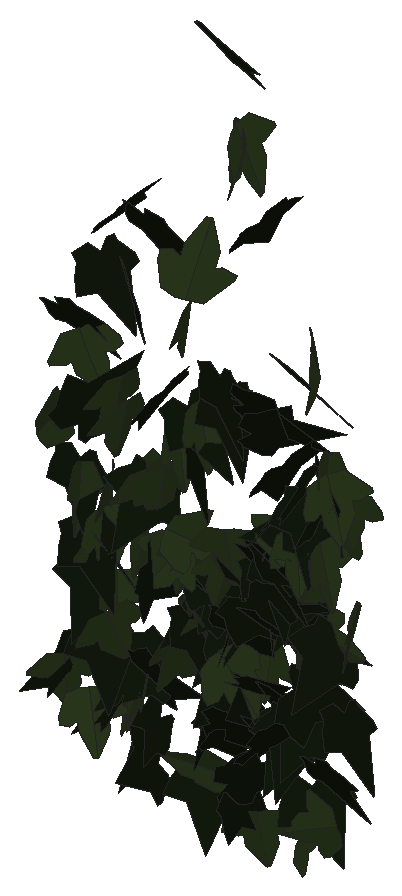
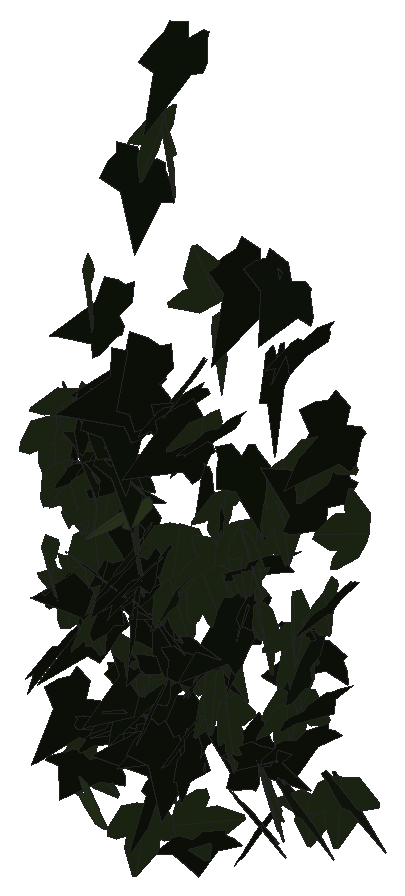
# SketchUp Ruby script. Lengths in inches.
U = 1.inch
M = Sketchup.active_model
def pt(a) = Geom::Point3d.new(a.map { |v| v * U })
def face(e, loops, mat)
  f = e.add_face(loops[0].map { |a| pt(a) })
  loops[1..].each { |l| e.add_face(l.map { |a| pt(a) }).erase! }
  f.material = f.back_material = mat if mat
  f
end
# faces: each face lists its corners as indices into pts; further lists are holes
def faces(e, pts, list, mat = nil) = list.each { |f| face(e, (f[0].is_a?(Array) ? f : [f]).map { |l| l.map { |i| pts[i] } }, mat) }
# xy, xz, yz: faces in a plane at the given z, y or x. An outline is a flat list of corners, or four numbers for a rectangle; further outlines are holes
def ring(l) = l.size == 4 ? [[l[0], l[1]], [l[2], l[1]], [l[2], l[3]], [l[0], l[3]]] : l.each_slice(2).to_a
def flat(e, list, mat, &to3) = list.each { |f| face(e, (f[0].is_a?(Array) ? f : [f]).map { |l| ring(l).map { |u, v| to3.(u, v) } }, mat) }
def xy(e, z, list, mat = nil) = flat(e, list, mat) { |x, y| [x, y, z] }
def xz(e, y, list, mat = nil) = flat(e, list, mat) { |x, z| [x, y, z] }
def yz(e, x, list, mat = nil) = flat(e, list, mat) { |y, z| [x, y, z] }
def lines(e, pts, list) = list.each { |a, b| e.add_line(pt(pts[a]), pt(pts[b])) }
# prism: a flat outline (further loops are holes) pulled along v
def prism(e, loops, v, mat = nil)
  f = face(e, loops, mat); d = Geom::Vector3d.new(v.map { |x| x * U })
  f.pushpull(f.normal.samedirection?(d) ? d.length : -d.length)
end
def box(e, o, s, mat = nil) = prism(e, [[o, [o[0] + s[0], o[1], o[2]], [o[0] + s[0], o[1] + s[1], o[2]], [o[0], o[1] + s[1], o[2]]]], [0, 0, s[2]], mat)
def at(x, y, z, deg = 0) = Geom::Transformation.translation(pt([x, y, z])) * Geom::Transformation.rotation(ORIGIN, Z_AXIS, deg.degrees)
def axes(o, x, y, z) = Geom::Transformation.new([*x, 0, *y, 0, *z, 0, *pt(o).to_a, 1])
def part(name) = M.definitions.add(name)
# library, detail: a bought-in or finely detailed component or shape, given as its bounding box
def library(name, o, s) = part(name).tap { |d| box(d.entities, o, s) }
def detail(e, o, s) = box(e.add_group.entities, o, s)
def put(e, d, t, mat = nil) = e.add_instance(d, t).tap { |i| i.material = mat if mat }
def group(e, t, mat = nil) = e.add_group.tap { |g| g.transformation = t; g.material = mat if mat }.entities
root = M.entities
M.materials.add("efeu1").color = [18, 25, 13]
M.materials.add("efeu2").color = [43, 57, 29]
c1 = part("ivyleaf_9")
p = [[1.54,2.16,1.25],[1.36,2.04,1.19],[-0.21,0.99,0.68],[-0.71,1.11,0.82],[-0.85,0.86,0.67],[-0.8,0.17,0.21],
  [-0.9,-0.01,0.1],[-0.67,-0.16,-0.02],[-0.08,-0.08,-0.05],[-0.03,-0.6,-0.4],[0.65,-0.88,-0.66],[0.83,-0.6,-0.49],
  [1.29,-0.42,-0.43],[1.8125,-0.07,-0.26],[1.21,0.44,0.15]]
faces(c1.entities,p,[[0,1,2,3,4,5,6,7,8,9,10,11,12,13,14]],"efeu1")
c2 = part("ivyleaf_10")
p = [[0,0.5,-0.03],[-0.0625,2.02,-0.43],[-0.19,2.01,-0.46],[-0.54,1.05,-0.29],[-0.52,0.625,-0.18],[-0.83,0.76,-0.28],
  [-1.16,0.64,-0.33],[-1.15,0.33,-0.24],[-0.77,-0.39,0.02],[-0.3,-0.51,0.16],[0.04,-0.48,0.23],[-0.02,2.01,-0.4375],
  [-0.06,2.01,-0.43],[0.04,-0.49,0.23],[0.67,-0.49,0.14],[1.38,0.36,-0.2],[1.375,0.51,-0.24],[0.81,0.65,-0.19],
  [0.62,0.59,-0.15],[0.6,1.09,-0.28],[0.5,1.23,-0.31]]
faces(c2.entities,p,[[0,1,2,3,4,5,6,7,8,9,10],[11,12,0,13,14,15,16,17,18,19,20]],"efeu2")
put(root,c1,axes([577.06,128.89,247.8],[-0.79782,0.64432,0.02333],[-0.05599,-0.03226,-1.02374],[-0.64231,-0.79751,0.06026]))
put(root,c2,axes([576.92,128.93,247.56],[-0.7328,-0.71537,-0.04037],[0.0378,0.01907,-1.02401],[0.71551,-0.73367,0.01274]))
put(root,c2,axes([576.88,128.08,257.89],[0.12693,-0.46512,1.05499],[-0.17832,1.04067,0.48026],[-1.1391,-0.21474,0.04237]))
put(root,c1,axes([576.91,129.79,255.57],[0.15146,-1.05206,0.06443],[0.00604,-0.06422,-1.0629],[1.05401,0.15154,-0.00316]))
put(root,c1,axes([576.97,128.67,262.52],[1.0872,0.15846,-0.03375],[-0.03824,0.02847,-1.09817],[-0.15743,1.08735,0.03367]))
put(root,c2,axes([577.51,129.17,255.4],[-0.09441,0.97241,-0.40538],[-0.04382,-0.41028,-0.97395],[-1.05261,-0.07014,0.0769]))
put(root,c1,axes([577.68,129.9375,251.1],[-0.32025,-0.94857,0.31634],[0.01052,-0.33535,-0.99491],[0.99987,-0.30029,0.11179]))
put(root,c2,axes([577.79,128.96,261.32],[-0.6989,-0.79219,-0.30752],[0.4449,-0.00187,-1.0063],[0.72401,-0.76356,0.32152]))
put(root,c2,axes([578.26,129.79,255.1],[0.37186,-0.92594,-0.35762],[-0.00755,0.37924,-0.98978],[0.99258,0.34978,0.12645]))
put(root,c2,axes([578.33,129.57,252.96],[-0.17488,-1.04729,0.05785],[0.19474,-0.09005,-1.0415],[1.03065,-0.16069,0.20661]))
put(root,c1,axes([577.74,129.77,252.8],[0.73564,-0.65,0.38792],[0.27873,-0.27032,-0.98152],[0.70377,0.78649,-0.01675]))
put(root,c1,axes([577.98,129.01,253.44],[-0.45566,-0.41074,-0.91799],[0.81737,0.43592,-0.60076],[0.58593,-0.92752,0.12417]))
put(root,c2,axes([578.2,128.71,246.47],[0.89283,0.43868,0.24577],[0.23293,0.08302,-0.9944],[-0.44563,0.92231,-0.02738]))
put(root,c1,axes([579.09,129.2,246.96],[-0.84178,0.56961,-0.05662],[0.04864,-0.02914,-1.01639],[-0.57035,-0.84318,-0.00312]))
put(root,c2,axes([578.53,129.26,253.82],[0.29311,1.02348,0.03769],[-0.06124,0.05665,-1.06202],[-1.02234,0.29004,0.07442]))
put(root,c1,axes([578.3125,128.08,258.54],[-0.13621,-0.13847,1.15186],[0.95976,0.63812,0.1902],[-0.65179,0.96858,0.03936]))
put(root,c2,axes([578.56,129.98,250.9],[0.095,1.01006,-0.29537],[0.00689,-0.29716,-1.01397],[-1.05234,0.08924,-0.0333]))
put(root,c1,axes([578.57,129.33,249.22],[-0.18032,-1.0131,-0.20221],[0.07323,0.19222,-1.02834],[1.03049,-0.19094,0.03769]))
put(root,c2,axes([579.3125,129.29,258.75],[-0.17827,-1.06893,-0.03979],[-0.02023,0.0437,-1.08336],[1.06948,-0.17735,-0.02713]))
put(root,c2,axes([579.32,129.06,259.875],[-0.15944,-1.08106,0.02862],[0.00294,-0.02937,-1.09273],[1.08144,-0.1593,0.00719]))
put(root,c1,axes([578.84,128.67,265.34],[0.30481,-0.93347,-0.48956],[-0.09061,0.48453,-0.98029],[1.05016,0.31275,0.05752]))
put(root,c2,axes([579.26,128.62,250.3],[-0.47944,-0.90072,-0.37557],[0.20089,0.31839,-1.02004],[0.95498,-0.51917,0.02602]))
put(root,c1,axes([579.86,128.95,264.28],[0.45779,0.08634,-1.10755],[-1.10437,0.16518,-0.4436],[0.12039,1.187,0.14229]))
put(root,c1,axes([579.61,128.51,267.49],[0.29425,0.92645,0.52974],[-0.03106,0.55671,-0.95636],[-1.06676,0.23934,0.17397]))
put(root,c2,axes([579.47,129.82,247.13],[0.75626,-0.72269,0.01223],[-0.00289,-0.02073,-1.04591],[0.72279,0.75608,-0.01699]))
put(root,c2,axes([579.7,129.77,247.4375],[0.80947,-0.66459,0.01205],[0.00806,-0.00917,-1.04734],[0.66465,0.8095,-0.00197]))
put(root,c1,axes([580.34,130.08,248.33],[-0.92376,-0.37392,0.24336],[-0.22806,-0.08518,-0.99654],[0.38344,-0.95147,-0.00642]))
put(root,c2,axes([580.13,129.28,253.89],[0.85893,-0.58825,-0.24217],[-0.0937,0.28548,-1.02575],[0.62921,0.84552,0.17785]))
put(root,c1,axes([580.53,129.82,245.99],[-0.93245,0.00042,-0.43465],[0.43123,-0.12795,-0.92524],[-0.05444,-1.0208,0.11579]))
put(root,c1,axes([580.58,129.61,255.86],[-0.6201,-0.82302,0.29027],[0.01548,-0.3664,-1.00581],[0.87257,-0.57839,0.22412]))
put(root,c1,axes([581.04,129.39,260.05],[-0.33209,1.01356,-0.1565],[0.02718,-0.15574,-1.06634],[-1.02521,-0.33244,0.02243]))
put(root,c1,axes([580.62,129.58,244.3125],[-0.28381,-0.40205,0.91877],[-0.15346,-0.92619,-0.4527],[0.99107,-0.25855,0.193]))
put(root,c2,axes([580.82,129.35,256.7],[0.8085,-0.67201,-0.18203],[-0.12031,0.1399,-1.05088],[0.68575,0.81685,0.03024]))
put(root,c2,axes([580.85,128.8,256.76],[-0.39099,-0.992,-0.26862],[0.09799,0.25011,-1.06627],[1.02304,-0.40308,-0.00053]))
put(root,c1,axes([580.24,129.65,247.81],[0.36484,-0.29991,0.91578],[0.74932,-0.52741,-0.47124],[0.60591,0.83283,0.03135]))
put(root,c1,axes([580.86,128.76,267.54],[1.20109,0.17587,-0.44977],[-0.44958,-0.0331,-1.21352],[-0.17636,1.28212,0.03037]))
put(root,c2,axes([581.18,129.99,249.74],[0.1389,-1.04108,-0.08736],[0.02626,0.09158,-1.04962],[1.04441,0.13615,0.03801]))
put(root,c1,axes([581.3125,128.31,253.44],[0.25462,-0.22787,-1.11533],[-0.84985,0.72234,-0.34159],[0.75739,0.88713,-0.00834]))
put(root,c2,axes([581.29,129.17,256.69],[-0.40381,-0.99757,-0.03403],[-0.00365,0.03818,-1.07606],[0.99815,-0.40344,-0.0177]))
put(root,c1,axes([580.98,129.7,253.25],[1.10341,-0.18849,-0.00836],[-0.00859,-0.00064,-1.1194],[0.18848,1.10345,-0.00208]))
put(root,c2,axes([581.65,129.71,258.41],[0.09464,1.06557,-0.0634],[-0.01788,-0.06206,-1.06969],[-1.0673,0.09553,0.0123]))
put(root,c2,axes([582.14,128.71,254.09],[0.91405,0.05653,-0.56273],[-0.56544,0.11302,-0.9071],[0.01146,1.06741,0.12585]))
put(root,c2,axes([582.1,129.82,250.87],[-0.90474,0.44109,0.26771],[-0.27617,0.0425,-1.00335],[-0.43584,-0.94256,0.08004]))
put(root,c2,axes([583.01,130.03,244.6],[-0.30018,0.16608,-0.97809],[-0.98382,-0.18152,0.27112],[-0.12785,1.00689,0.21021]))
put(root,c2,axes([582.55,129.51,254.28],[-0.28991,-0.98191,0.31894],[-0.04548,-0.31881,-1.02284],[1.03141,-0.29006,0.04455]))
put(root,c1,axes([582.99,130.12,251.95],[-1.03943,-0.02307,0.01489],[-0.01517,0.01257,-1.03961],[0.02289,-1.03946,-0.01291]))
put(root,c2,axes([582.62,128.57,250.34],[-0.14334,-0.9298,-0.828],[0.17778,0.80964,-0.93996],[1.23228,-0.22496,0.03929]))
put(root,c2,axes([582.78,128.67,264.4],[0.41347,-1.00666,-0.21323],[0.00175,0.23049,-1.08474],[1.02899,0.40411,0.08753]))
put(root,c1,axes([582.51,130.36,244.21],[-0.41387,-0.8742,-0.30009],[0.212,0.23025,-0.96312],[0.89963,-0.45643,0.08891]))
put(root,c1,axes([582.29,129.56,258.34],[-0.27173,-0.01761,-1.03792],[1.03789,0.01554,-0.27199],[0.0195,-1.07279,0.01309]))
put(root,c1,axes([582.5,129.3,251.09],[0.42187,-0.94909,-0.08441],[-0.03216,0.07808,-1.03862],[0.95229,0.42308,0.00232]))
put(root,c2,axes([582.54,128.58,254.9375],[0.33371,0.3441,0.95667],[0.47417,0.838,-0.46681],[-0.89933,0.56952,0.10886]))
put(root,c1,axes([582.89,130.375,247.69],[-0.1635,0.09515,-1.0236],[0.80095,-0.63795,-0.18724],[-0.64444,-0.81702,0.02699]))
put(root,c1,axes([583.1,130.58,247.94],[-0.1825,-0.64065,0.78184],[-0.07454,-0.78379,-0.65964],[1.00805,-0.17394,0.09277]))
put(root,c2,axes([583.1,128.43,265.83],[0.73989,0.84599,-0.48301],[0.3262,0.35637,1.12384],[0.91793,-0.80854,-0.01004]))
put(root,c1,axes([582.86,128.73,260.29],[0.40345,-0.89232,-0.45673],[0.02712,0.50187,-0.95656],[1.00205,0.34569,0.20978]))
put(root,c2,axes([583.73,129.98,253.85],[-0.28699,-0.98923,0.23334],[-0.01998,-0.23693,-1.02901],[1.01618,-0.28404,0.04567]))
put(root,c2,axes([583.5,128.71,260.25],[0.14802,1.07471,0.00521],[-0.00575,0.00605,-1.08483],[-1.0747,0.14799,0.00652]))
put(root,c1,axes([584.15,130.3125,251.17],[-0.89848,-0.50276,0.04313],[-0.04288,-0.0117,-1.02953],[0.50278,-0.89944,-0.01072]))
put(root,c1,axes([583.625,129,259.91],[0.55669,0.6289,0.69898],[0.47305,0.51468,-0.83983],[-0.81259,0.73046,-0.01005]))
put(root,c1,axes([584.13,128.8125,275.97],[1.01169,0.35803,-0.70253],[-0.78327,0.32487,-0.96239],[-0.09069,1.18807,0.47487]))
put(root,c1,axes([584.33,129.3,247.21],[0.27982,0.98286,-0.06512],[-0.03251,-0.05844,-1.02181],[-0.98448,0.28129,0.01523]))
put(root,c1,axes([584.13,130.39,252.45],[-0.39958,0.05698,-0.9592],[0.8047,-0.54789,-0.36777],[-0.52514,-0.88292,0.16631]))
put(root,c1,axes([583.68,129.97,253.89],[0.73557,-0.75627,0.08125],[0.13031,0.01394,-1.04997],[0.74938,0.73991,0.10283]))
put(root,c2,axes([584.45,128.96,255.35],[-0.97093,-0.47407,-0.06035],[0.05132,0.03245,-1.08047],[0.47513,-0.97227,-0.00663]))
put(root,c1,axes([584.01,129.09,261.76],[0.45563,-0.97493,0.12419],[0.04159,-0.11764,-1.07608],[0.98193,0.45737,-0.01205]))
put(root,c1,axes([584.58,130.32,252.67],[-0.88058,-0.12919,-0.52249],[0.53236,-0.0616,-0.88199],[0.07923,-1.02206,0.1192]))
put(root,c1,axes([583.98,128.69,247.65],[0.99081,0.19349,0.34196],[0.33382,0.07469,-1.00948],[-0.20722,1.04549,0.00883]))
put(root,c1,axes([584.29,129.3,261.07],[0.11435,-1.05858,-0.20086],[-0.0339,0.19836,-1.06467],[1.07694,0.11865,-0.01218]))
put(root,c2,axes([584.48,128.89,250.08],[0.55426,0.87957,0.5498],[0.22772,0.50497,-1.03743],[-1.01196,0.59539,0.06767]))
put(root,c2,axes([585.21,128.69,271.97],[0.50559,-0.82129,-0.7829],[-0.41238,0.66549,-0.96443],[1.05707,0.65243,-0.00178]))
put(root,c1,axes([584.81,130.19,248.22],[-0.12339,-0.38649,0.96478],[-0.11085,-0.96112,-0.3992],[1.03339,-0.14925,0.07238]))
put(root,c1,axes([585.17,128.61,245.24],[0.31343,-0.39065,-0.97171],[-0.61076,0.75578,-0.50085],[0.85077,0.68649,-0.00157]))
put(root,c1,axes([585.07,128.625,252.47],[1.05621,0.4368,-0.28002],[-0.25891,-0.10666,-1.14297],[-0.44963,1.08748,0.00037]))
put(root,c2,axes([585.27,128.85,272.35],[-0.12275,1.16093,0.32077],[-0.05871,0.31628,-1.16715],[-1.20299,-0.13389,0.02423]))
put(root,c2,axes([585.52,129.52,243.69],[-0.86853,-0.58891,-0.0854],[0.07563,0.04063,-1.04933],[0.59024,-0.87177,0.00879]))
put(root,c2,axes([585.51,129.94,255.35],[0.62998,-0.85151,-0.01828],[0.07467,0.07787,-1.05387],[0.84843,0.62541,0.10632]))
put(root,c1,axes([585.54,129.14,249.6],[0.92485,0.35972,-0.30435],[-0.36334,0.11756,-0.96516],[-0.30002,0.96651,0.23066]))
put(root,c1,axes([585.09,130.48,252.79],[0.06626,-0.00026,-1.0344],[0.9848,-0.3171,0.06317],[-0.31646,-0.98682,-0.02002]))
put(root,c1,axes([585.17,129.07,249.4375],[1.0613,0.27677,0.27272],[0.20706,0.26839,-1.07816],[-0.32879,1.06241,0.20132]))
put(root,c1,axes([585.3125,130.11,253.88],[0.34777,-0.96398,-0.24228],[-0.0021,0.25597,-1.02145],[0.99395,0.33783,0.08261]))
put(root,c2,axes([585.68,129.8,250.65],[1.01778,-0.15175,-0.03007],[-0.00333,0.17855,-1.01386],[0.15466,1.00245,0.17603]))
put(root,c1,axes([585.41,127.97,245.89],[0.4295,0.2747,0.93557],[0.79359,0.49551,-0.50981],[-0.56654,0.90235,-0.00486]))
put(root,c1,axes([585.48,129.09,255.1875],[1.04904,0.08714,0.11459],[0.11593,-0.0117,-1.05244],[-0.08534,1.05521,-0.02114]))
put(root,c1,axes([585.68,129.55,254.78],[1.05542,0.1427,-0.16912],[-0.16501,-0.0416,-1.06485],[-0.14743,1.06807,-0.01888]))
put(root,c1,axes([585.85,130.26,254.16],[0.14809,-1.02702,0.11184],[0.01306,-0.11111,-1.03764],[1.03301,0.14864,-0.00292]))
put(root,c1,axes([586.59,128.19,269.64],[0.06067,1.11423,0.15178],[0.00548,0.1517,-1.11587],[-1.1245,0.06086,0.00275]))
put(root,c1,axes([585.87,128.55,253.4],[-0.09701,-0.13846,-1.08358],[0.42376,0.99789,-0.16545],[1.00685,-0.43333,-0.03477]))
put(root,c1,axes([585.91,129.46,254.89],[0.70056,-0.78526,0.03083],[0.05944,0.01176,-1.05105],[0.78361,0.70114,0.05216]))
put(root,c1,axes([585.59,128.75,261.33],[1.01534,-0.20811,0.64502],[0.6316,-0.13089,-1.03644],[0.24585,1.19575,-0.00119]))
put(root,c1,axes([586.45,130.46,247.49],[-0.25145,-0.98898,0.18704],[-0.00311,-0.19202,-1.01951],[1.0065,-0.24767,0.04357]))
put(root,c1,axes([586.48,128,247.79],[0.47519,0.66369,0.75251],[0.32822,0.684,-0.81053],[-0.94817,0.5694,0.09655]))
put(root,c2,axes([586.13,129.09,256.16],[0.75807,-0.66906,-0.29363],[0.62188,0.81294,-0.24683],[0.38357,0.00428,0.98051]))
put(root,c1,axes([586.74,130.41,247.8],[-0.7456,-0.72291,-0.02914],[0.14093,-0.10407,-1.02405],[0.70964,-0.73888,0.17275]))
put(root,c1,axes([587.21,128.45,257.47],[-0.17083,1.00321,0.31999],[-0.14901,0.29788,-1.01344],[-1.04241,-0.20698,0.09243]))
put(root,c1,axes([586.13,128.5,260.56],[0.75911,0.30787,0.82494],[0.74037,0.36638,-0.81803],[-0.47661,1.0595,0.04316]))
put(root,c1,axes([587.4,128.53,259.6],[-0.04557,1.09241,-0.10476],[0.02756,-0.10368,-1.09312],[-1.09708,-0.04798,-0.02311]))
put(root,c1,axes([587.41,130.5,253.88],[-0.95436,-0.18504,-0.36514],[0.39814,-0.20428,-0.93708],[0.09515,-1.00119,0.25868]))
put(root,c2,axes([587.65,129.78,254.41],[-0.97496,0.00075,0.3707],[-0.37003,-0.06486,-0.97306],[0.02235,-1.04104,0.0609]))
put(root,c2,axes([587.31,129.45,256.04],[0.451,0.94161,-0.02503],[-0.01393,-0.02108,-1.04404],[-0.94184,0.4512,0.00346]))
put(root,c1,axes([588.22,129.6875,256.84],[-0.21286,-0.32121,-0.99616],[-0.55577,-0.82672,0.38533],[-0.88692,0.59514,-0.00238]))
put(root,c1,axes([588.08,128.85,258.8],[-0.74346,0.73663,-0.22142],[0.08207,-0.23021,-1.04146],[-0.76479,-0.74078,0.10347]))
put(root,c2,axes([587.57,129.86,251.55],[-0.09183,0.939,-0.42122],[0.0128,-0.42182,-0.94312],[-1.02907,-0.08904,0.02585]))
put(root,c2,axes([587.32,129.88,243.31],[0.31596,-0.77769,-0.65248],[0.56347,-0.43408,0.79022],[-0.84442,-0.58064,0.28316]))
put(root,c2,axes([588.45,129.54,251.76],[-0.89327,-0.10422,0.56888],[-0.53986,-0.2252,-0.88896],[0.20745,-1.03482,0.13617]))
put(root,c1,axes([587.26,129.7,252.49],[0.22627,0.09525,-1.03432],[0.80175,0.65699,0.2359],[0.66037,-0.83029,0.068]))
put(root,c2,axes([587.64,129.78,256.12],[-0.13818,0.15546,-1.04467],[0.46748,-0.93575,-0.20109],[-0.94708,-0.48457,0.05316]))
put(root,c1,axes([587.66,129.99,245.53],[-0.24405,-0.71089,-0.71488],[0.47684,0.56666,-0.72629],[0.88828,-0.49951,0.19347]))
put(root,c1,axes([587.35,128.84,263.54],[0.90915,-0.54833,0.2968],[0.33262,-0.01732,-1.05089],[0.52737,0.95621,0.15116]))
put(root,c1,axes([587.95,129.63,257.61],[-0.18978,-1.04973,-0.09161],[0.00893,0.09148,-1.06672],[1.05368,-0.18984,-0.00745]))
put(root,c2,axes([588.97,129.11,244.82],[-0.39798,0.03149,0.95846],[-0.93561,-0.24041,-0.3806],[0.21039,-1.00957,0.12053]))
put(root,c1,axes([588.07,128.46,250.47],[0.44067,-0.05563,-1.07306],[-0.43966,1.04893,-0.23493],[0.98043,0.49538,0.37695]))
put(root,c2,axes([588.85,129.91,256.83],[-0.87,-0.20003,0.54473],[-0.52637,-0.14123,-0.89254],[0.24429,-1.0167,0.01681]))
put(root,c1,axes([589.02,128.61,257.94],[-0.27708,0.87515,0.55939],[-0.24436,0.50778,-0.91544],[-1.00951,-0.36312,0.06806]))
put(root,c2,axes([589,128.36,264.18],[0.15361,-0.32446,-1.20122],[-0.58234,1.05085,-0.35831],[1.09958,0.60186,-0.02196]))
put(root,c2,axes([588.77,129.5,259.6],[-0.15086,0.95695,-0.45403],[0.01541,-0.45658,-0.96745],[-1.05909,-0.14296,0.0506]))
put(root,c2,axes([588.21,129.8125,252.42],[-0.19891,0.09621,-1.0405],[0.98128,-0.34687,-0.21966],[-0.35917,-1.00095,-0.02389]))
put(root,c1,axes([588.41,129.76,258.11],[0.08334,-0.2082,1.04216],[0.3779,-0.97123,-0.22425],[0.99329,0.38698,-0.00212]))
put(root,c1,axes([589.06,129.53,252.17],[-0.48845,-0.86812,0.31716],[-0.1911,-0.25611,-0.99533],[0.90427,-0.52305,-0.03902]))
put(root,c1,axes([588.68,129.03,247.22],[1.05306,0.05494,-0.12972],[-0.12952,-0.00719,-1.05449],[-0.05541,1.06099,-0.00043]))
put(root,c2,axes([589,128.91,256.18],[-0.05103,1.0448,0.0032],[0.00346,0.00337,-1.04604],[-1.0448,-0.05102,-0.00362]))
put(root,c2,axes([589.55,129.64,258.32],[-0.93755,-0.4727,0.04378],[-0.03212,-0.03353,-1.04987],[0.47364,-0.93798,0.01546]))
put(root,c2,axes([589.48,130.06,253.28],[0.57456,-0.85291,0.23371],[0.16097,-0.17319,-1.02776],[0.86958,0.59561,0.03583]))
put(root,c2,axes([589.49,128.68,259.28],[0.53365,0.91545,0.1932],[0.04711,0.19584,-1.05811],[-0.93443,0.53269,0.05699]))
put(root,c1,axes([589.49,129.54,249.4],[0.39003,-0.9262,-0.29678],[-0.09913,0.28023,-1.00483],[0.96752,0.40208,0.01669]))
